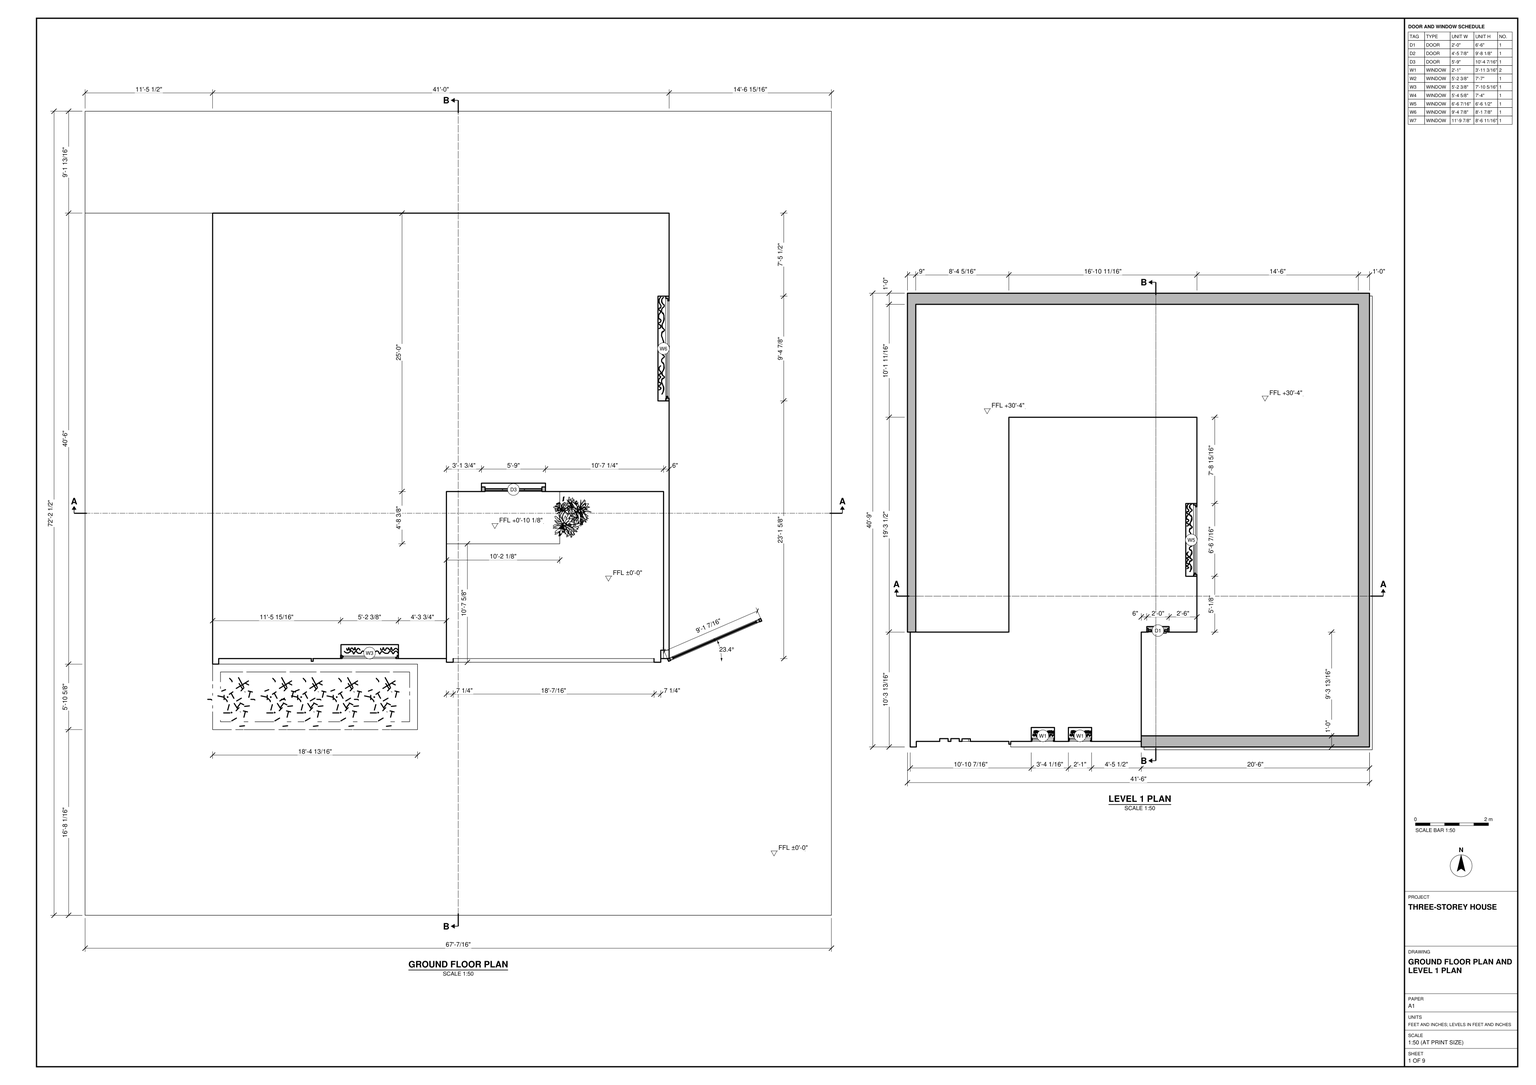
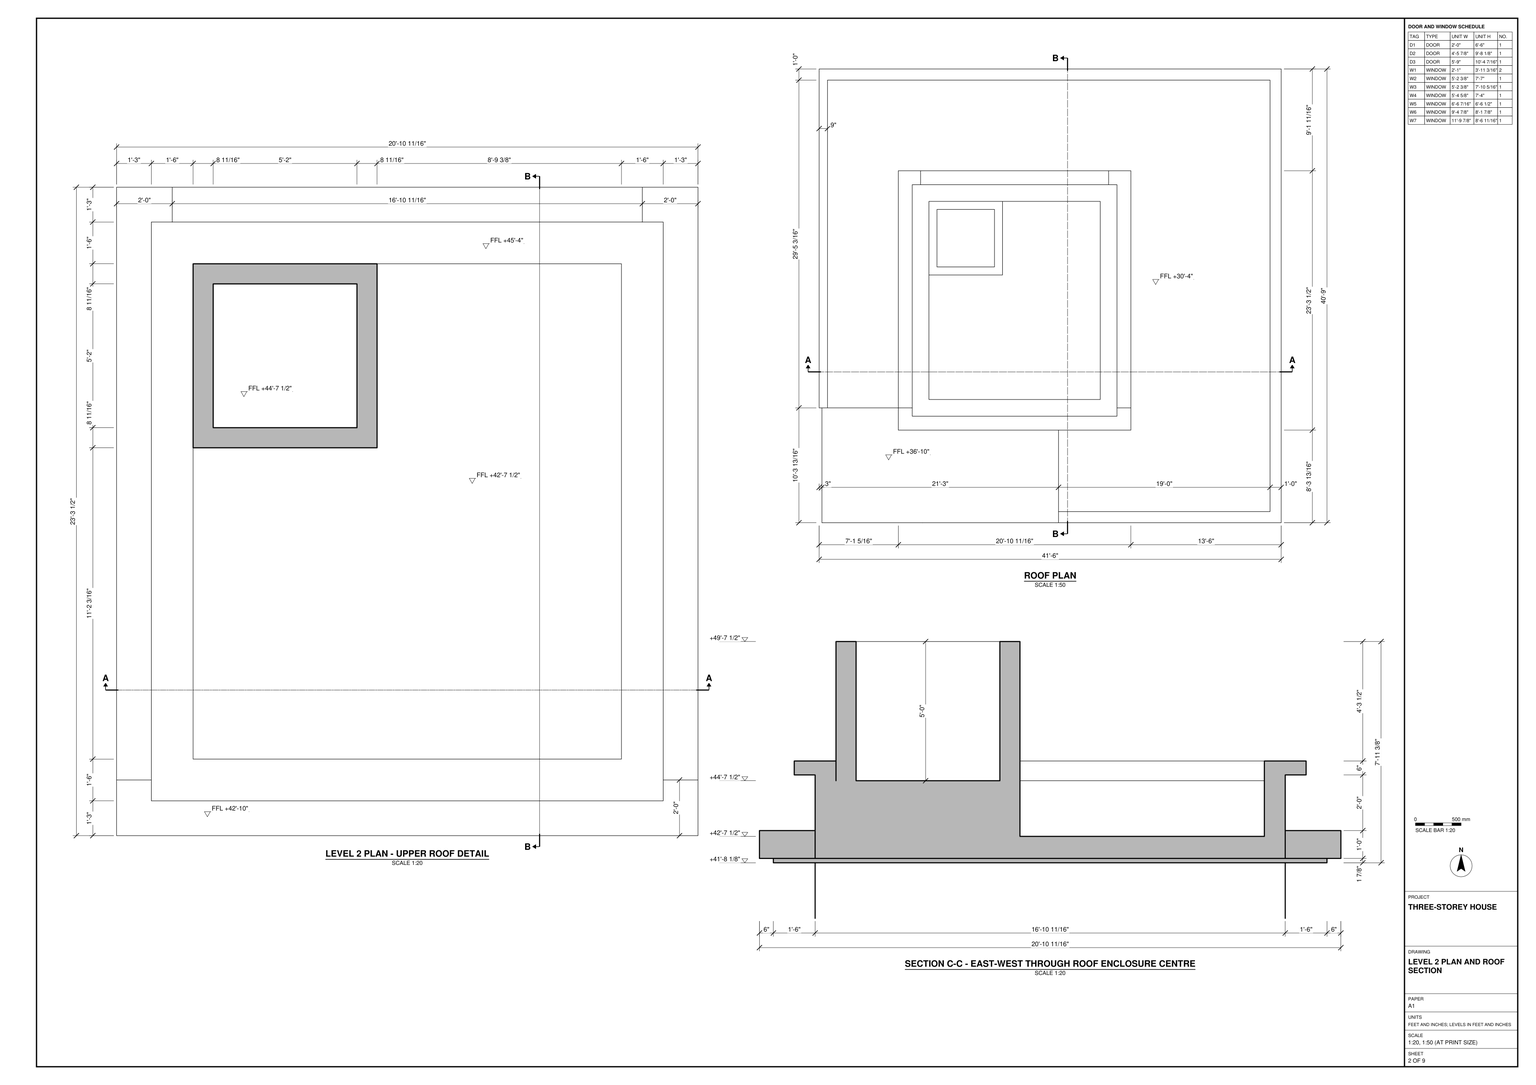
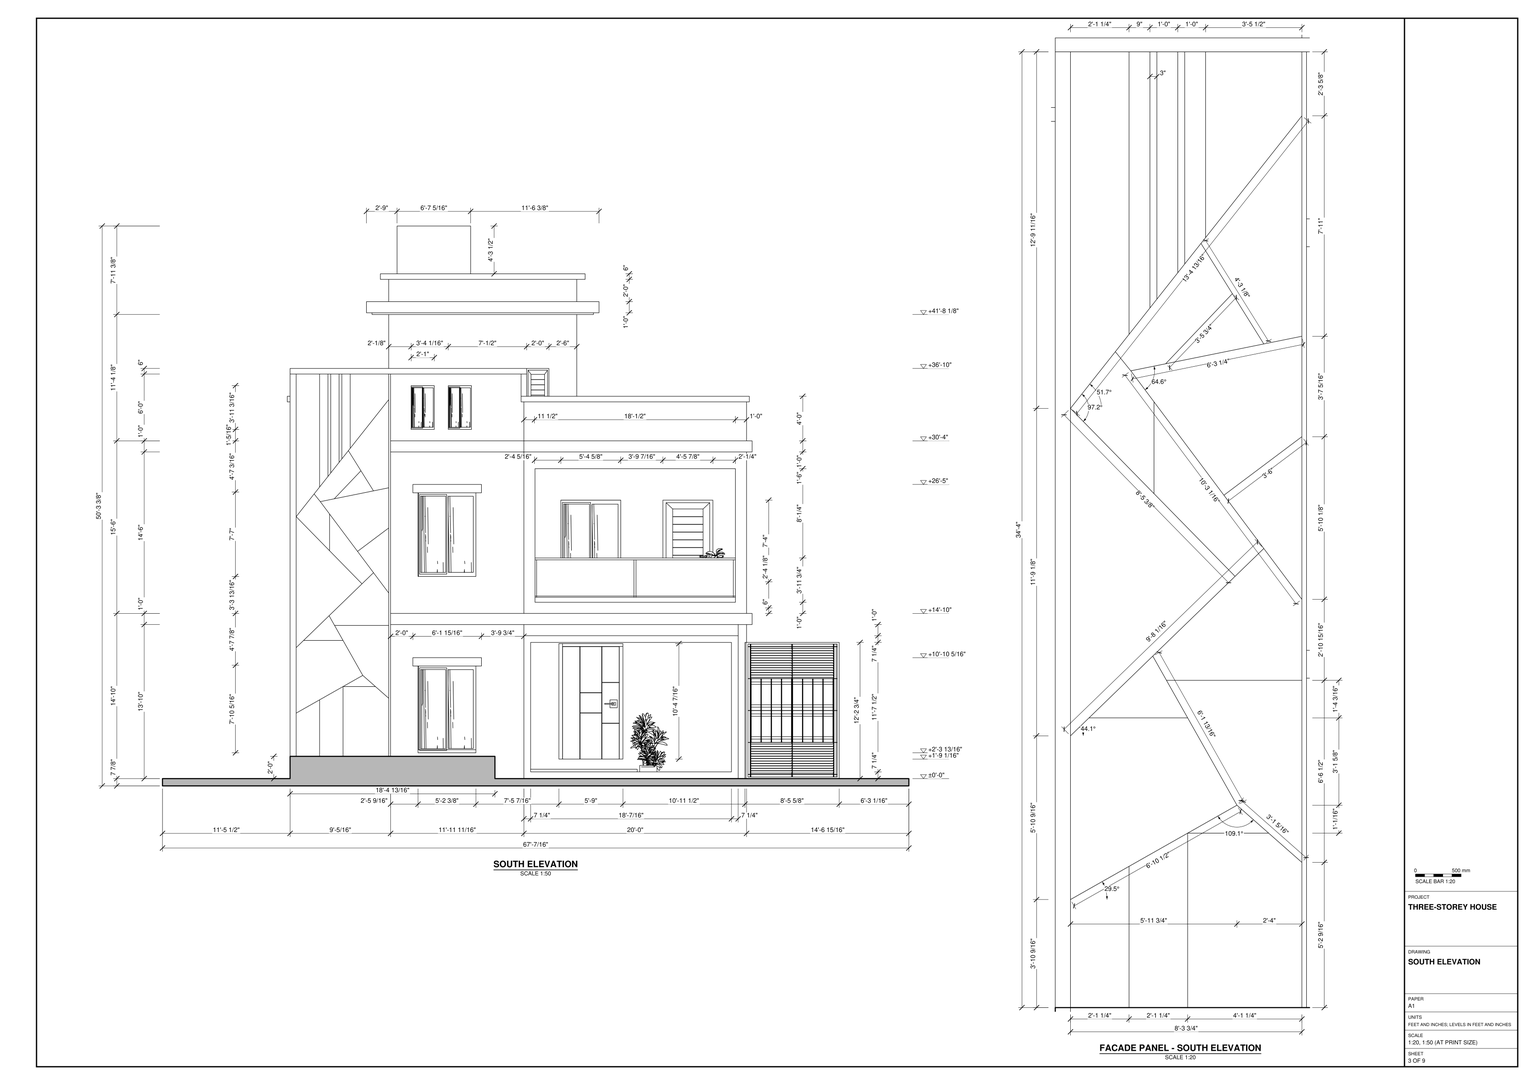
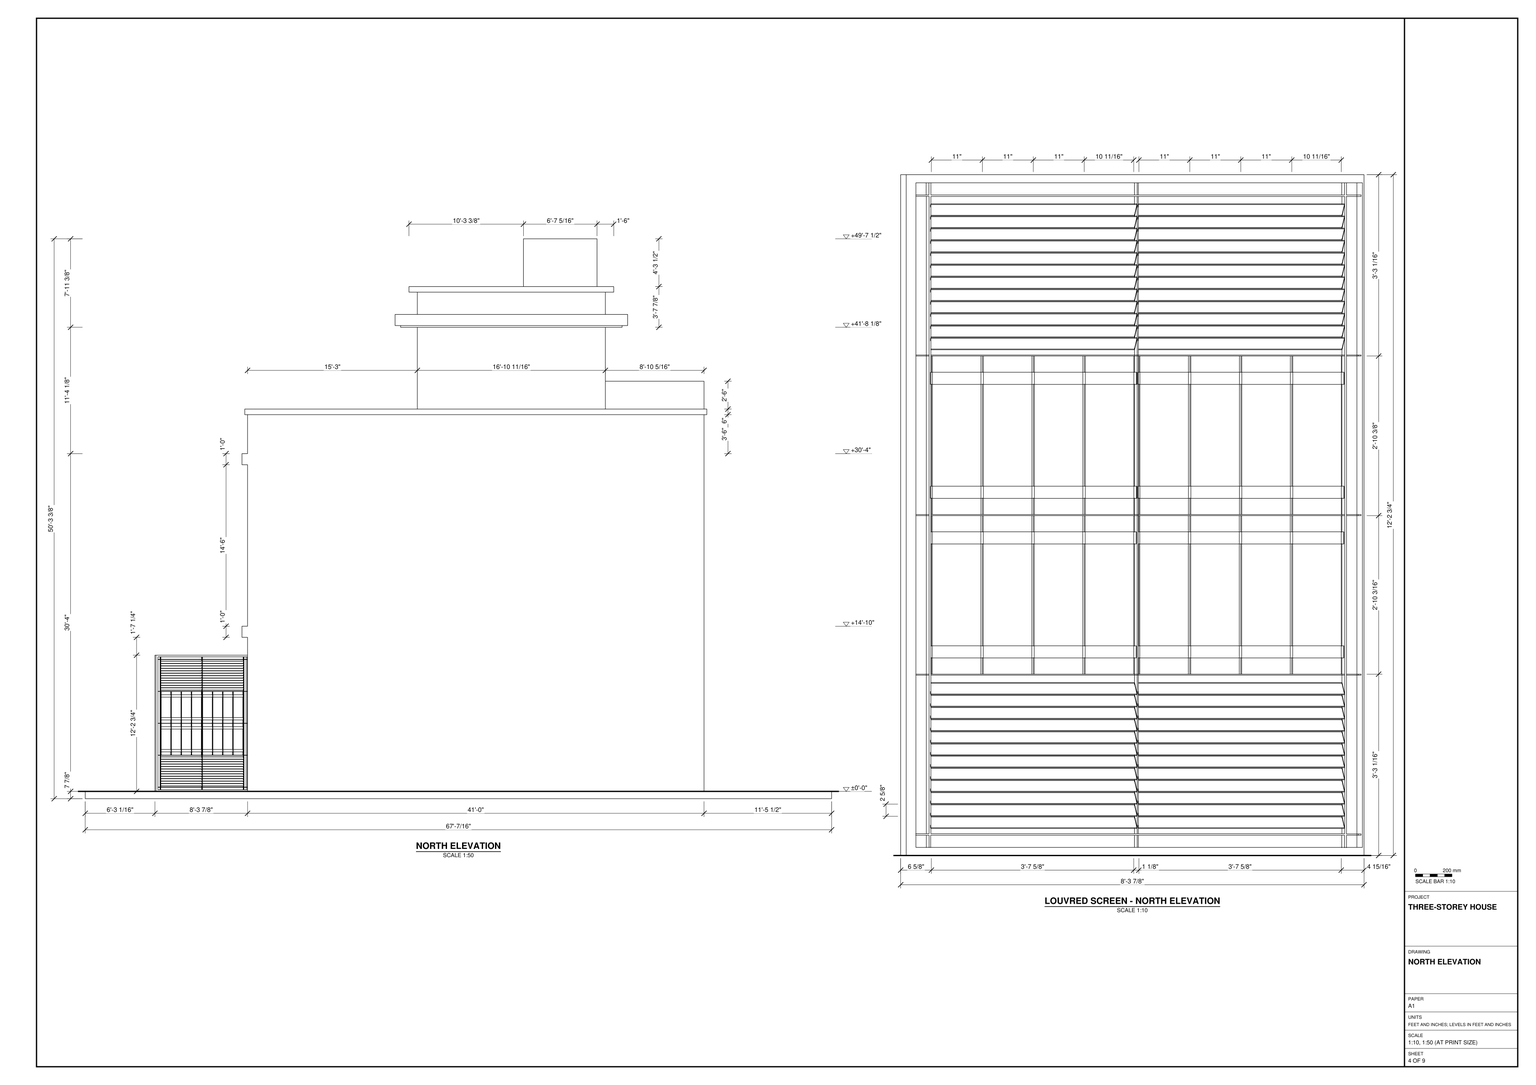
Build the three-storey house in SketchUp from task_files/diagram_01.pdf. Work in feet and inches. Including the rectangular site slab, the overall model must measure 67'-7/16" along X, 72'-2 1/2" along Y and 50'-3 3/8" along Z. Use the storey levels ±0'-0", +30'-4" and +41'-8 1/8" relative to the ground floor.

Use the plans to position the house on the slab and to set out the wall thicknesses, setbacks and openings. On the south elevation, recess the entrance beneath the balcony and fit the balcony with its panelled glass railing. Use the enlarged facade detail to lay out the diagonal and vertical divisions of the tall panel on the left. Set the slatted gate to the right of the entrance at the angle shown in plan. Match the doors and windows to the schedule and elevations. Follow the roof plan and section to model the projecting slab edges, parapets and raised square enclosure. Include stairs, built-in joinery and main furniture where shown.

Keep shell elements such as walls, slabs and roofs, and each furniture or joinery piece, in separate groups or components. Use components for repeated parts. Decor and loose items, including plants, may be any suitable library components. Save one SketchUp model as output_files/three_storey_house_with_its_balcony_and_stepped_roof.skp.

# SketchUp Ruby script. Lengths in inches.
U = 1.inch
M = Sketchup.active_model
def pt(a) = Geom::Point3d.new(a.map { |v| v * U })
def face(e, loops, mat)
  f = e.add_face(loops[0].map { |a| pt(a) })
  loops[1..].each { |l| e.add_face(l.map { |a| pt(a) }).erase! }
  f.material = f.back_material = mat if mat
  f
end
# faces: each face lists its corners as indices into pts; further lists are holes
def faces(e, pts, list, mat = nil) = list.each { |f| face(e, (f[0].is_a?(Array) ? f : [f]).map { |l| l.map { |i| pts[i] } }, mat) }
# xy, xz, yz: faces in a plane at the given z, y or x. An outline is a flat list of corners, or four numbers for a rectangle; further outlines are holes
def ring(l) = l.size == 4 ? [[l[0], l[1]], [l[2], l[1]], [l[2], l[3]], [l[0], l[3]]] : l.each_slice(2).to_a
def flat(e, list, mat, &to3) = list.each { |f| face(e, (f[0].is_a?(Array) ? f : [f]).map { |l| ring(l).map { |u, v| to3.(u, v) } }, mat) }
def xy(e, z, list, mat = nil) = flat(e, list, mat) { |x, y| [x, y, z] }
def xz(e, y, list, mat = nil) = flat(e, list, mat) { |x, z| [x, y, z] }
def yz(e, x, list, mat = nil) = flat(e, list, mat) { |y, z| [x, y, z] }
def lines(e, pts, list) = list.each { |a, b| e.add_line(pt(pts[a]), pt(pts[b])) }
# prism: a flat outline (further loops are holes) pulled along v
def prism(e, loops, v, mat = nil)
  f = face(e, loops, mat); d = Geom::Vector3d.new(v.map { |x| x * U })
  f.pushpull(f.normal.samedirection?(d) ? d.length : -d.length)
end
def box(e, o, s, mat = nil) = prism(e, [[o, [o[0] + s[0], o[1], o[2]], [o[0] + s[0], o[1] + s[1], o[2]], [o[0], o[1] + s[1], o[2]]]], [0, 0, s[2]], mat)
def at(x, y, z, deg = 0) = Geom::Transformation.translation(pt([x, y, z])) * Geom::Transformation.rotation(ORIGIN, Z_AXIS, deg.degrees)
def axes(o, x, y, z) = Geom::Transformation.new([*x, 0, *y, 0, *z, 0, *pt(o).to_a, 1])
def part(name) = M.definitions.add(name)
# library, detail: a bought-in or finely detailed component or shape, given as its bounding box
def library(name, o, s) = part(name).tap { |d| box(d.entities, o, s) }
def detail(e, o, s) = box(e.add_group.entities, o, s)
def put(e, d, t, mat = nil) = e.add_instance(d, t).tap { |i| i.material = mat if mat }
def group(e, t, mat = nil) = e.add_group.tap { |g| g.transformation = t; g.material = mat if mat }.entities
root = M.entities
M.materials.add("Glass Railing Color").color = [198, 198, 198]
M.materials.add("Railing Glass").color = [63, 150, 137]
M.materials["Railing Glass"].alpha = 0.13
M.materials.add("[0030_OldLace]1").color = [221, 214, 201]
M.materials.add("[0035_Tan]").color = [190, 177, 159]
M.materials.add("[0036_BurlyWood]").color = [139, 135, 125]
M.materials.add("[0057_DarkKhaki]1").color = [144, 142, 120]
M.materials.add("[0134_DimGray]").color = [105, 105, 105]
M.materials.add("[0136_Charcoal]").color = [35, 35, 35]
M.materials.add("[Blacktop Old 02]").color = [226, 229, 229]
M.materials.add("[Polished Concrete New]").color = [223, 223, 226]
M.materials.add("[Stone Sandstone Ashlar Light]").color = [206, 178, 128]
M.materials.add("[Wood Veneer 01]").color = [120, 70, 37]
M.materials.add("hymenocallis littoralis").color = [156, 172, 146]
c1 = library("window",[15.03,5.62,-3.05],[94.49,12.1,85.64])
c2 = library("door (4)",[38.93,25.48,0],[40,9.94,82.68])
c3 = library("Door+80x210",[17.88,40.74,0],[31.52,6.14,82.69])
c4 = library("Wade+gate+5.2",[0,-3,0],[48,3,84])
c5 = part("Glass Rail Spacer")
box(c5.entities,[-0.5,-0.25,0],[1,0.5,1],"Glass Railing Color")
c6 = part("Group138\#1")
prism(c6.entities,[[[0.54,0,1.27],[0.38,0,1.39],[0.21,0,1.47],[0.01,0,1.5],[-0.18,0,1.48],[-0.37,0,1.41],[-0.52,0,1.29],[-0.64,0,1.13],[-0.72,0,0.96],[-0.75,0,0.76],[-0.73,0,0.57],[-0.66,0,0.38],[-0.54,0,0.23],[-0.38,0,0.11],[-0.21,0,0.03],[-0.01,0,0],[0.18,0,0.02],[0.37,0,0.09],[0.52,0,0.21],[0.64,0,0.37],[0.72,0,0.54],[0.75,0,0.74],[0.73,0,0.93],[0.66,0,1.12]]],[0,97,0],"Glass Railing Color")
c7 = part("Group141\#1")
prism(c7.entities,[[[0.25,0,5],[0.25,0,4],[-0.25,0,4],[-0.25,0,5],[-0.5,0,5],[-0.5,0,0],[0.5,0,0],[0.5,0,5]]],[0,97,0],"Glass Railing Color")
c8 = part("Group144\#1")
box(c8.entities,[-0.1875,0,0],[0.375,47,30],"Railing Glass")
c9 = part("Group147\#1")
box(c9.entities,[-0.1875,0,0],[0.375,47,30],"Railing Glass")
c10 = part("Glass Railing\#8")
put(c10.entities,c5,at(0,0,4))
put(c10.entities,c5,at(48,0,4))
put(c10.entities,c5,at(96,0,4))
put(c10.entities,c6,at(-0.5,0,34,-90))
put(c10.entities,c7,at(-0.5,0,0,-90))
put(c10.entities,c8,at(0.5,0,4,-90))
put(c10.entities,c9,at(48.5,0,4,-90))
c11 = library("Group_2",[-1.28,-0.39,0],[21.22,20.51,48.44])
c12 = library("plant (7)",[-35.72,-28.42,0],[66.31,67.39,84.38])
c13 = part("Group\#856")
xy(c13.entities,7.38,[[0,0,5.5,15.91]],"hymenocallis littoralis")
p = [[5.5,28.78,0],[5.5,26.79,3.44],[0,26.79,3.44],[0,28.78,0],[0,23.75,6],[5.5,23.75,6],
  [0,15.91,7.38],[5.5,15.91,7.38]]
faces(c13.entities,p,[[0,1,2,3],[4,2,1,5],[6,4,5,7]],"hymenocallis littoralis")
c14 = part("Group\#854")
xy(c14.entities,7.38,[[0,0,5.5,15.91],[0,15.91,5.5,23.87]],"hymenocallis littoralis")
p = [[5.5,31.07,4.3],[5.5,27.74,6.47],[0,27.74,6.47],[0,31.07,4.3],[0,23.87,7.38],[5.5,23.87,7.38]]
faces(c14.entities,p,[[0,1,2,3],[4,2,1,5]],"hymenocallis littoralis")
c15 = part("Group\#857")
xy(c15.entities,7.38,[[0,0,5.6,15.91]],"hymenocallis littoralis")
p = [[5.6,28.78,0],[5.6,26.79,3.44],[0,26.79,3.44],[0,28.78,0],[0,23.75,6],[5.6,23.75,6],
  [0,15.91,7.38],[5.6,15.91,7.38]]
faces(c15.entities,p,[[0,1,2,3],[4,2,1,5],[6,4,5,7]],"hymenocallis littoralis")
c16 = part("Group\#855")
put(c16.entities,c14,axes([6.09,8.57,-0.52],[0.446,0.85617,0.26089],[-0.18444,-0.19731,0.96283],[0.87582,-0.47754,0.0699]))
put(c16.entities,c14,axes([6.29,7.28,-1.71],[0.37058,0.92707,-0.05667],[-0.32382,0.19004,0.99128],[0.87712,-0.32925,0.34964]))
put(c16.entities,c14,axes([11.04,16.14,-0.7],[1,0,0],[0,0.16628,1.02662],[0,-1.18456,0.19186]))
c17 = part("Group\#860")
put(c17.entities,c13,axes([24.57,32.05,-1.76],[0.9552,-0.22102,-0.19681],[0.4036,0.95545,0.88585],[-0.00568,-0.67859,0.7345]))
put(c17.entities,c13,axes([23.95,29.24,-2.4],[0,1,0],[-0.76041,0,0.64945],[0.64945,0,0.76041]))
put(c17.entities,c13,axes([24.22,24.72,-0.48],[-0.70711,0.70711,0],[-0.32757,-0.32757,0.80237],[0.61237,0.61237,0.5]))
put(c17.entities,c14,axes([20.66,37.22,-0.63],[1.12361,0.03262,0.39091],[-0.43499,0.29739,0.78777],[0.09852,-1.27434,0.37535]))
put(c17.entities,c13,axes([28.75,24.45,-2.4],[-1,0,0],[0,-0.76041,0.64945],[0,0.64945,0.76041]))
put(c17.entities,c15,axes([30.4,30.98,-3.7],[0.65676,-0.72002,0.22414],[0.55667,0.66341,0.5],[-0.50871,-0.20361,0.83652]))
put(c17.entities,c15,axes([32.41,29.61,-3.7],[0.04029,-0.97372,0.22414],[0.85287,0.15038,0.5],[-0.52057,0.17102,0.83652]))
put(c17.entities,c13,axes([31.89,25.85,-1.76],[-0.92056,0.33739,-0.19681],[-0.5186,-0.89824,0.88585],[0.08952,0.67268,0.7345]))
put(c17.entities,c13,axes([25.55,34.78,-0.48],[0.86603,0.5,0],[-0.25,0.43301,0.86603],[0.43301,-0.75,0.5]))
put(c17.entities,c15,axes([20.4,16.9375,-8.07],[-0.70711,0.70711,0],[-0.35754,-0.35754,0.65422],[1.3987,1.3987,1.52882]))
put(c17.entities,c13,axes([32.86,34.14,-0.48],[0.76604,-0.64279,0],[0.32139,0.38302,0.86603],[-0.55667,-0.66341,0.5]))
put(c17.entities,c13,axes([27.15,34.7,-0.1],[0.82472,-0.17528,-0.53769],[0.53769,0.53769,0.64945],[0.17528,-0.82472,0.53769]))
put(c17.entities,c13,axes([33.58,28.77,-2.4],[0,-1,0],[0.76041,0,0.64945],[-0.64945,0,0.76041]))
put(c17.entities,c13,axes([26.43,23.87,-2.81],[-0.75126,0.04415,0.65853],[0.53769,-0.53769,0.64945],[0.38276,0.84199,0.3802]))
put(c17.entities,c13,axes([28.78,23.98,-2.4],[-1,0,0],[0,-0.76041,0.64945],[0,0.64945,0.76041]))
put(c17.entities,c13,axes([25.39,25.38,-2.4],[-0.70711,0.70711,0],[-0.53769,-0.53769,0.64945],[0.45923,0.45923,0.76041]))
put(c17.entities,c13,axes([27.32,21.63,-0.1],[-0.45923,0.70711,-0.53769],[-0.76041,0,0.64945],[0.45923,0.70711,0.53769]))
put(c17.entities,c13,axes([25.17,27.625,-1.76],[0.56416,0.80187,-0.19681],[-0.66673,0.66673,0.80532],[0.62659,-0.26057,0.7345]))
put(c17.entities,c15,axes([27.59,27.04,-3.96],[-0.8993,-0.06127,0.43301],[0.2962,-0.8138,0.5],[0.32175,0.57791,0.75]))
put(c17.entities,c15,axes([26.98,24.5,-3.18],[-0.5,0.86603,0],[-0.75,-0.43301,0.5],[0.43301,0.25,0.86603]))
put(c17.entities,c15,axes([24.55,27.74,-3.7],[0.29517,0.92878,0.22414],[-0.85287,0.15038,0.5],[0.43068,-0.33875,0.83652]))
put(c17.entities,c15,axes([24.26,29.8,-3.18],[0.76604,0.64279,0],[-0.47317,0.5639,0.425],[0.32139,-0.38302,0.86603]))
put(c17.entities,c15,axes([25.98,32.46,-3.18],[1,0,0],[0,0.86603,0.5],[0,-0.5,0.86603]))
put(c17.entities,c13,axes([28.78,33.57,-2.4],[1,0,0],[0,0.76041,0.64945],[0,-0.64945,0.76041]))
put(c17.entities,c16,at(14.99,21.38,2.5))
put(c17.entities,c14,axes([34.63,26.34,-1.46],[-0.70089,-0.70877,0.07994],[0.4756,-0.38088,0.79293],[-0.53156,0.59378,0.60405]))
put(c17.entities,c14,axes([28.14,16.92,1.8125],[-1.19719,0.6912,0],[-0.09607,-0.16641,0.94244],[0.68444,1.18549,0.17613]))
put(c17.entities,c14,axes([31.5625,35.84,0.97],[0.66765,-1.1564,0.35779],[0.04445,0.30732,0.91033],[-1.20828,-0.64496,0.17012]))
put(c17.entities,c14,axes([38.94,22.51,0.89],[-0.97932,-0.67164,-0.05202],[0.27787,-0.41401,0.90999],[-0.85985,0.93577,0.32097]))
put(c17.entities,c14,axes([38.44,21.09,1.98],[-1.02864,-0.54856,0.2395],[0.33481,0.06999,0.88388],[-0.77261,1.08328,0.06417]))
put(c17.entities,c15,axes([35.02,30.51,-1.3],[-0.17365,-0.98481,0],[0.60224,-0.10619,0.79122],[-0.7792,0.13739,0.61153]))
put(c17.entities,c15,axes([29.41,22.33,-1.3],[-0.93969,0.34202,0],[-0.20915,-0.57465,0.79122],[0.27061,0.74351,0.61153]))
put(c17.entities,c14,axes([19.64,36,-1.62],[1.18194,0.09546,0.08234],[-0.14377,0.68823,0.76313],[0.21457,-1.1326,0.62386]))
put(c17.entities,c15,axes([24.25,24.14,-1.3],[-0.34202,0.93969,0],[-0.57465,-0.20915,0.79122],[0.74351,0.27061,0.61153]))
put(c17.entities,c15,axes([25.98,34.61,-1.3],[1,0,0],[0,0.61153,0.79122],[0,-0.79122,0.61153]))
put(c17.entities,c15,axes([31.16,34.41,-1.64],[0.56518,-0.80224,-0.19234],[0.73413,0.34233,0.72935],[-0.47639,-0.50772,0.71782]))
put(c17.entities,c15,axes([40.52,26.84,-5.82],[-0.42262,-0.90631,0],[0.48019,-0.22391,0.68552],[-1.43418,0.66877,1.22305]))
put(c17.entities,c13,axes([29.86,38.42,-1.01],[0.89064,-0.37013,0.26413],[-0.03924,0.63286,1.01918],[-0.45353,-0.76487,0.45748]))
put(c17.entities,c13,axes([29.34,22.4,-0.48],[-0.99619,-0.08716,0],[0.04358,-0.4981,0.86603],[-0.07548,0.86273,0.5]))
c18 = part("Group\#858")
xz(c18.entities,10.07,[[9.07,0,10.07,31.01],[0,31.01,0,45.12,20.13,45.12,20.13,31.01,10.07,31.01,10.07,32.58,9.07,32.58,9.07,31.01]],"hymenocallis littoralis")
yz(c18.entities,10.07,[[0,31.01,20.13,45.12]],"hymenocallis littoralis")
p = [[9.57,9.2,0],[10.07,10.07,0],[10.07,10.07,31.01],[10.07,10.07,32.58],[9.57,9.2,32.58]]
faces(c18.entities,p,[[0,1,2,3,4]],"hymenocallis littoralis")
c19 = part("cây lá nắng")
put(c19.entities,c17,axes([49.26,-2.75,0],[0.63109,0.63109,0],[-0.63109,0.63109,0],[0,0,0.935]))
g1 = group(c19.entities,at(26.6,-8.68,0))
put(g1,c13,axes([-4.72,35.73,-1.65],[0.74231,0.46334,-0.18402],[-0.34827,0.85768,0.82827],[0.42467,-0.43184,0.68675]))
put(g1,c13,axes([-3.34,33.57,-2.24],[-0.63109,0.63109,0],[-0.47989,-0.47989,0.60723],[0.40986,0.40986,0.71098]))
put(g1,c13,axes([-0.3125,30.89,-0.45],[-0.8925,0,0],[0,-0.41345,0.75022],[0,0.77293,0.4675]))
put(g1,c14,axes([-10.79,39.66,-0.59],[0.68852,0.72969,0.3655],[-0.4622,-0.08684,0.73657],[0.86641,-0.74205,0.35095]))
put(g1,c13,axes([2.71,33.57,-2.24],[-0.63109,-0.63109,0],[0.47989,-0.47989,0.60723],[-0.40986,0.40986,0.71098]))
put(g1,c15,axes([-0.37,38.74,-3.46],[0.86887,-0.03992,0.20957],[-0.06737,0.76999,0.4675],[-0.19255,-0.44954,0.78214]))
put(g1,c15,axes([1.76,39.14,-3.46],[0.63993,-0.58908,0.20957],[0.44333,0.63315,0.4675],[-0.43646,-0.2206,0.78214]))
put(g1,c13,axes([3.81,36.4375,-1.65],[-0.79389,-0.36803,-0.18402],[0.23959,-0.89415,0.82827],[-0.36803,0.48102,0.68675]))
put(g1,c13,axes([-5.83,38.07,-0.45],[0.231,0.86209,0],[-0.43104,0.1155,0.80973],[0.74659,-0.20005,0.4675]))
put(g1,c15,axes([2.18,23.5625,-7.55],[-0.8925,0,0],[0,-0.45128,0.6117],[0,1.76542,1.42944]))
put(g1,c13,axes([-0.8125,42.28,-0.45],[0.8891,0.07779,0],[-0.03889,0.44455,0.80973],[0.06737,-0.76999,0.4675]))
put(g1,c13,axes([-4.76,39.03,-0.09],[0.63109,0.40986,-0.50274],[0,0.67866,0.60723],[0.63109,-0.40986,0.50274]))
put(g1,c13,axes([3.03,39.35,-2.24],[0.63109,-0.63109,0],[0.47989,0.47989,0.60723],[-0.40986,-0.40986,0.71098]))
put(g1,c13,axes([1.61,31.74,-2.625],[-0.50198,-0.44625,0.61573],[0.67866,0,0.60723],[-0.28982,0.77293,0.35549]))
put(g1,c13,axes([3.03,33.3,-2.24],[-0.63109,-0.63109,0],[0.47989,-0.47989,0.60723],[-0.40986,0.40986,0.71098]))
put(g1,c13,axes([0.01,32.04,-2.24],[-0.8925,0,0],[0,-0.67866,0.60723],[0,0.57963,0.71098]))
put(g1,c13,axes([3.59,30.89,-0.09],[-0.73607,0.15643,-0.50274],[-0.47989,-0.47989,0.60723],[-0.15643,0.73607,0.50274]))
put(g1,c13,axes([-1.55,33.32,-1.65],[-0.15002,0.86209,-0.18402],[-0.84154,0,0.75297],[0.55988,0.231,0.68675]))
put(g1,c15,axes([0.35,34.48,-3.71],[-0.52887,-0.60621,0.40487],[0.70051,-0.32665,0.4675],[-0.16166,0.56777,0.70125]))
put(g1,c15,axes([2.61,39.13,-1.74],[-0.86209,0.231,0],[-0.23031,-0.85954,0.15531],[0.03162,0.11799,0.91645]))
put(g1,c15,axes([-2.02,33,-3.46],[-0.39986,0.77243,0.20957],[-0.63315,-0.44333,0.4675],[0.48558,0.05802,0.78214]))
put(g1,c15,axes([-3.49,34.12,-2.97],[0.07779,0.8891,0],[-0.65449,0.05726,0.39737],[0.44455,-0.03889,0.80973]))
put(g1,c15,axes([-4.09,36.88,-2.97],[0.63109,0.63109,0],[-0.54654,0.54654,0.4675],[0.31555,-0.31555,0.80973]))
put(g1,c13,axes([-3.02,39.35,-2.24],[0.63109,0.63109,0],[-0.47989,0.47989,0.60723],[0.40986,-0.40986,0.71098]))
put(g1,c16,axes([-4.03,22.95,2.33],[0.63109,0.63109,0],[-0.63109,0.63109,0],[0,0,0.935]))
put(g1,c14,axes([5.24,38.48,-1.37],[0.00497,-0.88963,0.07474],[0.54052,0.05978,0.74139],[-0.71019,0.03927,0.56479]))
put(g1,c14,axes([7.08,28.4375,1.7],[-1.19175,-0.31933,0],[0.04439,-0.16565,0.88118],[-0.31621,1.1801,0.16468]))
put(g1,c14,axes([-2.7,42.54,0.91],[1.15114,-0.30845,0.33454],[-0.1659,0.22199,0.85115],[-0.3555,-1.16957,0.15907]))
put(g1,c14,axes([10.37,38.78,0.83],[-0.19417,-1.04191,-0.04864],[0.43664,-0.08592,0.85084],[-1.1332,0.04791,0.30011]))
put(g1,c14,axes([10.95,37.5625,1.85],[-0.30298,-0.99536,0.22393],[0.16713,0.25547,0.82643],[-1.17124,0.19607,0.06]))
put(g1,c15,axes([2.84,41.36,-1.22],[0.51192,-0.73109,0],[0.44708,0.31305,0.73979],[-0.57846,-0.40504,0.57178]))
put(g1,c15,axes([4.47,32.65,-1.22],[-0.80888,-0.37719,0],[0.23066,-0.49465,0.73979],[-0.29844,0.64,0.57178]))
put(g1,c14,axes([-10.32,35.12,-1.51],[0.68567,0.80616,0.07699],[-0.52507,0.3436,0.71352],[0.85019,-0.57936,0.58331]))
put(g1,c15,axes([0.07,30.54,-1.22],[-0.80888,0.37719,0],[-0.23066,-0.49465,0.73979],[0.29844,0.64,0.57178]))
put(g1,c15,axes([-5.45,38.24,-1.22],[0.63109,0.63109,0],[-0.38593,0.38593,0.73979],[0.49934,-0.49934,0.57178]))
put(g1,c15,axes([-2.05,41.38,-1.53],[0.86296,-0.14961,-0.17984],[0.24726,0.67935,0.68194],[0.01977,-0.62107,0.67116]))
put(g1,c15,axes([8.63,42.51,-5.4375],[0.30525,-0.83868,0],[0.44435,0.16173,0.64096],[-1.32716,-0.48305,1.14356]))
put(g1,c13,axes([-5.4,43.09,-0.94],[0.79566,0.32849,0.24696],[-0.42416,0.37462,0.95293],[0.19648,-0.76892,0.42774]))
put(g1,c13,axes([4.38,32.65,-0.45],[-0.57369,-0.68369,0],[0.34185,-0.28684,0.80973],[-0.5921,0.49683,0.4675]))
put(g1,c15,axes([-2,33.84,-0.15],[-0.24601,0.85793,0],[-0.85539,-0.24528,0.15531],[0.11742,0.03367,0.91645]))
put(g1,c15,axes([0.17,30.83,-4.47],[-0.24601,0.85793,0],[-0.85539,-0.24528,0.15531],[0.11742,0.03367,0.91645]))
put(g1,c15,axes([-1.97,32.18,-4.47],[0.58524,0.67383,0],[-0.67184,0.58351,0.15531],[0.09222,-0.0801,0.91645]))
put(g1,c15,axes([-2,34.71,-4.47],[0.88392,-0.12346,0],[0.12309,0.88131,0.15531],[-0.0169,-0.12098,0.91645]))
put(g1,c15,axes([0.11,36.12,-4.47],[0.37822,-0.8084,0],[0.80601,0.37711,0.15531],[-0.11064,-0.05177,0.91645]))
put(c19.entities,c18,axes([29.71,14.29,6.94],[0.425,0.73612,0],[-0.6771,0.39092,-0.33349],[-0.26859,0.15507,0.72712]))
put(c19.entities,c18,axes([42.0625,26.12,6.94],[0.85,0,0],[0,0.78185,-0.33349],[0,0.33349,0.78185]))
put(c19.entities,c17,axes([7.3125,23.0625,0],[0.8925,0,0],[0,0.8925,0],[0,0,0.935]))
put(c19.entities,c18,axes([24.4375,40.23,2.05],[0.85,0,0],[0,0.85,0],[0,0,0.85]))
c20 = part("Planting+101")
put(c20.entities,c19,axes([21.34,32.96,-4.59],[0,-0.71,0],[-0.71,0,0],[0,0,0.71]))
xy(root,6.125,[[[0,0,804.4375,866.5],[620.5,276.6875,629.5,285.6875]],[620.5,276.6875,623.5,285.6875],[623.5,276.6875,629.5,285.6875]])
xy(root,13.99,[[145.98,208.54,349.84,262.21]],"[0030_OldLace]1")
xy(root,13.99,[[0,0,804.4375,0,804.4375,866.5,0,866.5,0,756.6875,629.5,756.6875,629.5,276.6875,620.5,276.6875,620.5,272.6875,389.5,272.6875,389.5,276.6875,245.83,276.6875,245.83,273.6875,243.83,273.6875,243.83,276.6875,144.0625,276.6875,144.0625,270.6875,358.3125,270.6875,358.3125,200.0625,137.5,200.0625,137.5,756.6875,0,756.6875],[389.5,272.6875,620.5,272.6875,620.5,276.6875,623.5,276.6875,623.5,456.6875,511.625,456.6875,511.625,400.3125,389.5,400.3125]],"[Polished Concrete New]")
xy(root,21.26,[[396.77,272.6875,613.23,276.6875]],"[0136_Charcoal]")
xy(root,24.11,[[389.5,400.3125,511.625,456.6875]],"[Wood Veneer 01]")
xy(root,35.04,[[427.24,456.6875,496.24,465.6875]])
xy(root,37.99,[[[137.5,200.0625,358.3125,270.6875],[145.98,208.54,349.84,262.21]]],"[0030_OldLace]1")
xy(root,39.84,[[617.5,554.34,629.5,667.21]])
xy(root,45.13,[[275.84,276.6875,337.77,291.6875]],"[0134_DimGray]")
xy(root,91,[[623.5,285.6875,629.5,382.5]],"[0030_OldLace]1")
xy(root,135.32,[[269.84,270.6875,269.84,276.6875,275.84,276.6875,275.84,291.6875,337.77,291.6875,337.77,276.6875,343.77,276.6875,343.77,270.6875]],"[0030_OldLace]1")
xy(root,137.65,[[617.5,554.34,629.5,667.21]])
xy(root,144.32,[[269.84,270.6875,343.77,276.6875]],"[0030_OldLace]1")
xy(root,159.48,[[427.24,456.6875,496.24,465.6875]])
xy(root,160.73,[[396.77,272.6875,613.23,276.6875]],"[0136_Charcoal]")
xy(root,168,[[389.5,276.6875,620.5,282.6875],[623.5,285.6875,629.5,382.5]],"[0030_OldLace]1")
xy(root,168,[[389.5,272.6875,620.5,276.6875]],"[0136_Charcoal]")
xy(root,180,[[389.5,282.6875,389.5,456.6875,623.5,456.6875,623.5,285.6875,620.5,285.6875,620.5,282.6875]],"[0030_OldLace]1")
xy(root,180,[[245.83,267.6875,389.5,276.6875],[389.5,267.6875,389.5,276.6875,629.5,276.6875,629.5,456.6875,635.5,456.6875,635.5,267.6875],[629.5,456.6875,635.5,756.6875]],"[0057_DarkKhaki]1")
xy(root,192,[[245.83,267.6875,635.5,267.6875,635.5,273.6875,389.5,273.6875,389.5,276.6875,245.83,276.6875],[629.5,273.6875,635.5,756.6875]],"[0057_DarkKhaki]1")
xy(root,198,[[395.5,282.6875,617.5,282.6875,617.5,336.6875,593.22,336.6875,593.22,345.6875,539.35,345.6875,539.35,336.6875,395.5,336.6875]],"[0030_OldLace]1")
xy(root,204,[[401.5,273.6875,617.5,282.6875],[617.5,282.6875,629.5,336.6875]],"[0030_OldLace]1")
xy(root,226.11,[[429.31,336.6875,493.93,351.6875]],"[0134_DimGray]")
xy(root,228.88,[[617.5,391.65,629.5,533.53]])
xy(root,231.82,[[275.84,276.6875,337.77,291.6875]],"[0134_DimGray]")
xy(root,314.11,[[539.35,336.6875,593.22,345.6875]])
xy(root,314.11,[[429.31,336.6875,493.93,351.6875]],"[0134_DimGray]")
xy(root,322,[[269.84,270.6875,269.84,276.6875,275.84,276.6875,275.84,291.6875,337.77,291.6875,337.77,276.6875,343.77,276.6875,343.77,270.6875]],"[0030_OldLace]1")
xy(root,331,[[269.84,270.6875,343.77,276.6875]],"[0030_OldLace]1")
xy(root,331.5,[[617.5,391.65,629.5,533.53]])
xy(root,348,[[401.5,273.6875,617.5,282.6875]],"[0030_OldLace]1")
xy(root,354,[[395.5,282.6875,629.5,336.6875]],"[0030_OldLace]1")
xy(root,366,[[389.5,267.6875,389.5,273.6875,629.5,273.6875,629.5,756.6875,635.5,756.6875,635.5,267.6875],[245.83,270.6875,389.5,276.6875]],"[0057_DarkKhaki]1")
xy(root,378,[[386.5,282.6875,620.5,282.6875,620.5,747.6875,143.5,747.6875,143.5,394.48,243.83,394.48,243.83,626,446.5,626,446.5,394.48,416.5,394.48,416.5,400.48,392.5,400.48,392.5,394.48,386.5,394.48]],"[0030_OldLace]1")
xy(root,378,[[389.5,267.6875,635.5,267.6875,635.5,756.6875,629.5,756.6875,629.5,273.6875,389.5,273.6875],[245.83,270.6875,389.5,276.6875]],"[0057_DarkKhaki]1")
xy(root,390.3,[[267.95,276.6875,292.95,291.6875],[308.01,276.6875,333.01,291.6875]],"[0134_DimGray]")
xy(root,398.3,[[434.5,454.61,446.5,533.05]])
xy(root,420,[[386.5,276.6875,389.5,282.6875]])
xy(root,420,[[386.5,270.6875,386.5,276.6875,389.5,276.6875,389.5,273.6875,629.5,273.6875,629.5,756.6875,137.5,756.6875,137.5,394.48,134.5,394.48,134.5,759.6875,632.5,759.6875,632.5,270.6875]],"[0057_DarkKhaki]1")
xy(root,426,[[386.5,270.6875,632.5,270.6875,632.5,759.6875,134.5,759.6875,134.5,394.48,143.5,394.48,143.5,747.6875,620.5,747.6875,620.5,282.6875,386.5,282.6875]],"[0057_DarkKhaki]1")
xy(root,437.42,[[267.95,276.6875,292.95,291.6875],[308.01,276.6875,333.01,291.6875]],"[0134_DimGray]")
xy(root,450,[[144.0625,270.6875,144.0625,276.6875,169.32,276.6875,169.32,279.6875,178.32,279.6875,178.32,276.6875,181.32,276.6875,181.32,279.6875,190.32,279.6875,190.32,276.6875,193.32,276.6875,193.32,279.5,202.32,279.5,202.32,276.6875,243.83,276.6875,243.83,270.6875],[243.83,270.6875,245.83,273.6875],[245.83,270.6875,245.83,276.6875,386.5,276.6875,386.5,394.48,392.5,394.48,392.5,270.6875]],"[0057_DarkKhaki]1")
xy(root,456,[[392.5,394.48,416.5,400.48]])
xy(root,456,[[137.5,270.6875,392.5,394.48]],"[0057_DarkKhaki]1")
xy(root,476.74,[[434.5,454.61,446.5,533.05]])
xy(root,514.125,[[243.83,394.48,446.5,626]])
xy(root,514.125,[[[225.83,376.48,464.5,644],[243.83,394.48,446.5,626]]],"[0030_OldLace]1")
xy(root,516,[[225.83,376.48,243.83,644],[243.83,376.48,464.5,394.48],[243.83,394.48,446.5,626],[446.5,394.48,464.5,626],[243.83,626,464.5,644]])
xy(root,516,[[[219.83,370.48,470.5,650],[225.83,376.48,464.5,644]]],"[0030_OldLace]1")
xy(root,525.5,[[252.83,403.48,437.5,403.48,437.5,617,332.14,617,332.14,537.6875,252.83,537.6875]],"[0030_OldLace]1")
xy(root,528,[[219.83,370.48,470.5,394.48],[219.83,394.48,243.83,650],[446.5,394.48,470.5,650],[243.83,626,446.5,650]],"[0030_OldLace]1")
xy(root,549.5,[[261.49,546.35,323.48,608.34]])
xy(root,552,[[[234.83,385.48,455.5,635],[243.83,394.48,446.5,626]]],"[0036_BurlyWood]")
xy(root,558,[[[234.83,385.48,455.5,635],[252.83,403.48,437.5,617]]],"[0036_BurlyWood]")
xy(root,609.5,[[[252.83,537.6875,332.14,617],[261.49,546.35,323.48,608.34]]],"[0035_Tan]")
xz(root,0,[[0,6.125,804.4375,13.99]],"[Blacktop Old 02]")
xz(root,200.0625,[[137.5,13.99,358.3125,37.99]],"[0030_OldLace]1")
xz(root,208.54,[[145.98,13.99,349.84,37.99]],"[0030_OldLace]1")
xz(root,262.21,[[145.98,13.99,349.84,37.99]],"[0030_OldLace]1")
xz(root,267.6875,[[245.83,180,635.5,192],[389.5,366,635.5,378]],"[0057_DarkKhaki]1")
xz(root,270.6875,[[144.0625,13.99,358.3125,37.99]])
xz(root,270.6875,[[269.84,135.32,343.77,144.32],[269.84,322,343.77,331]],"[0030_OldLace]1")
xz(root,270.6875,[[137.5,37.99,144.0625,450],[245.83,366,389.5,378],[386.5,420,632.5,426],[137.5,450,392.5,456]],"[0057_DarkKhaki]1")
xz(root,272.6875,[[[389.5,13.99,620.5,168],[396.77,21.26,613.23,160.73]]],"[0136_Charcoal]")
xz(root,273.6875,[[[389.5,192,629.5,366],[401.5,204,617.5,348]],[389.5,378,629.5,420]],"[0030_OldLace]1")
xz(root,273.6875,[[243.83,13.99,245.83,450]],"[0057_DarkKhaki]1")
xz(root,276.6875,[[620.5,6.125,623.5,13.99],[623.5,6.125,629.5,13.99]])
xz(root,276.6875,[[144.0625,13.99,169.32,13.99,169.32,98.88,144.0625,84.57],[169.32,13.99,194.58,13.99,194.58,113.1875,169.32,98.88],[194.58,13.99,243.83,13.99,243.83,100.58,229.51,113.1875,194.58,113.1875],[620.5,13.99,629.5,180],[243.83,100.58,243.83,179.06,185.45,179.06,194.58,162.88,215.84,125.23,229.51,113.1875],
  [144.0625,155.14,152.05,162.88,179.54,189.52,215.02,223.9,180.08,259.55,144.0625,296.29],[389.5,168,620.5,180],[185.45,179.06,243.83,179.06,243.83,213.98,227.41,235.9,215.02,223.9,179.54,189.52],[243.83,213.98,243.83,284.1,210.22,258.87,227.41,235.9],[215.02,223.9,227.41,235.9,210.22,258.87,180.08,299.12,180.08,259.55],
  [210.22,258.87,243.83,284.1,243.83,327.39,227.41,324.07,185.09,315.52,170.07,312.48,180.08,299.12],[144.0625,296.29,163.41,320.74,169.32,328.22,169.32,450,144.0625,450],[170.07,312.48,185.09,315.52,213.87,345.74,200.32,367.41,193.32,358.56,190.32,354.77,181.32,343.39,178.32,339.6,169.32,328.22,163.41,320.74],[227.41,324.07,243.83,327.39,243.83,422.39,202.32,369.93,200.32,367.41,213.87,345.74],[178.32,339.6,181.32,343.39,181.32,450,178.32,450],
  [190.32,354.77,193.32,358.56,193.32,450,190.32,450],[202.32,369.93,243.83,422.39,243.83,450,202.32,450],[[245.83,378,389.5,378,389.5,420,386.5,420,386.5,450,245.83,450],[267.95,390.3,292.95,437.42],[308.01,390.3,333.01,437.42]]],"[0030_OldLace]1")
xz(root,276.6875,[[[245.83,13.99,389.5,180],[275.84,45.13,275.84,135.32,269.84,135.32,269.84,144.32,343.77,144.32,343.77,135.32,337.77,135.32,337.77,45.13]],[144.0625,84.57,169.32,98.88,194.58,113.1875,215.84,125.23,194.58,162.88,152.05,162.88,144.0625,155.14]],"[0035_Tan]")
xz(root,276.6875,[[[245.83,192,389.5,366],[275.84,231.82,275.84,322,269.84,322,269.84,331,343.77,331,343.77,322,337.77,322,337.77,231.82]]],"[0036_BurlyWood]")
xz(root,276.6875,[[194.58,113.1875,229.51,113.1875,215.84,125.23],[152.05,162.88,194.58,162.88,185.45,179.06,179.54,189.52],[180.08,259.55,180.08,299.12,170.07,312.48,163.41,320.74,144.0625,296.29],[185.09,315.52,227.41,324.07,213.87,345.74]],"[0057_DarkKhaki]1")
xz(root,279.5,[[193.32,358.56,200.32,367.41,202.32,369.93,202.32,450,193.32,450]],"[0057_DarkKhaki]1")
xz(root,279.6875,[[169.32,328.22,178.32,339.6,178.32,450,169.32,450],[181.32,343.39,190.32,354.77,190.32,450,181.32,450]],"[0057_DarkKhaki]1")
xz(root,282.6875,[[389.5,168,620.5,180],[395.5,198,617.5,204],[395.5,204,401.5,354],[617.5,204,629.5,354],[401.5,348,617.5,354],
  [386.5,378,398.5,426],[398.5,378,620.5,426]],"[0030_OldLace]1")
xz(root,285.6875,[[623.5,6.125,629.5,13.99]])
xz(root,285.6875,[[620.5,6.125,623.5,180],[623.5,91,629.5,168]],"[0030_OldLace]1")
xz(root,291.6875,[[275.84,45.13,337.77,135.32],[275.84,231.82,337.77,322],[267.95,390.3,292.95,437.42],[308.01,390.3,333.01,437.42]],"[0134_DimGray]")
xz(root,336.6875,[[[395.5,198,539.35,198,539.35,314.11,593.22,314.11,593.22,198,617.5,198,617.5,204,629.5,204,629.5,354,395.5,354],[429.31,226.11,493.93,314.11]]],"[0030_OldLace]1")
xz(root,345.6875,[[539.35,198,593.22,314.11]])
xz(root,351.6875,[[429.31,226.11,493.93,314.11]],"[0134_DimGray]")
xz(root,370.48,[[219.83,516,470.5,528]],"[0030_OldLace]1")
xz(root,376.48,[[225.83,514.125,464.5,516]],"[0030_OldLace]1")
xz(root,382.5,[[623.5,91,629.5,168]],"[0030_OldLace]1")
xz(root,385.48,[[234.83,552,455.5,558]],"[0036_BurlyWood]")
xz(root,391.65,[[617.5,228.88,629.5,331.5]])
xz(root,394.48,[[137.5,420,143.5,426],[243.83,516,446.5,528]])
xz(root,394.48,[[143.5,378,143.5,426,137.5,426,137.5,456,243.83,456,243.83,378],[416.5,378,446.5,378,446.5,514.125,243.83,514.125,243.83,456,416.5,456],[386.5,378,392.5,450],[134.5,420,137.5,426]],"[0030_OldLace]1")
xz(root,394.48,[[243.83,528,446.5,552]],"[0036_BurlyWood]")
xz(root,400.3125,[[389.5,13.99,511.625,24.11]],"[Wood Veneer 01]")
xz(root,400.48,[[392.5,378,416.5,456]])
xz(root,403.48,[[252.83,525.5,437.5,549.5],[252.83,549.5,437.5,558]],"[0036_BurlyWood]")
xz(root,454.61,[[434.5,398.3,446.5,476.74]])
xz(root,456.6875,[[[511.625,13.99,623.5,13.99,623.5,180,389.5,180,389.5,24.11,511.625,24.11],[427.24,35.04,496.24,159.48]]],"[0030_OldLace]1")
xz(root,465.6875,[[427.24,35.04,496.24,159.48]])
xz(root,533.05,[[434.5,398.3,446.5,476.74]])
xz(root,533.53,[[617.5,228.88,629.5,331.5]])
xz(root,537.6875,[[252.83,525.5,332.14,609.5]],"[0035_Tan]")
xz(root,546.35,[[261.49,549.5,323.48,609.5]],"[0035_Tan]")
xz(root,554.34,[[617.5,39.84,629.5,137.65]])
xz(root,608.34,[[261.49,549.5,323.48,609.5]],"[0035_Tan]")
xz(root,617,[[252.83,549.5,332.14,558]])
xz(root,617,[[252.83,558,332.14,609.5]],"[0035_Tan]")
xz(root,617,[[332.14,525.5,437.5,549.5],[332.14,549.5,437.5,558]],"[0036_BurlyWood]")
xz(root,626,[[243.83,516,446.5,528]])
xz(root,626,[[243.83,378,446.5,514.125]],"[0030_OldLace]1")
xz(root,626,[[243.83,528,446.5,552]],"[0036_BurlyWood]")
xz(root,635,[[234.83,552,455.5,558]],"[0036_BurlyWood]")
xz(root,644,[[225.83,514.125,464.5,516]],"[0030_OldLace]1")
xz(root,650,[[219.83,516,470.5,528]],"[0030_OldLace]1")
xz(root,667.21,[[617.5,39.84,629.5,137.65]])
xz(root,747.6875,[[143.5,378,398.5,378,398.5,426,389.5,426,389.5,420,143.5,420],[398.5,378,620.5,426],[143.5,420,389.5,426]],"[0030_OldLace]1")
xz(root,756.6875,[[0,6.125,137.5,13.99],[137.5,6.125,629.5,13.99]])
xz(root,756.6875,[[137.5,13.99,137.5,420,629.5,420,629.5,378,635.5,378,635.5,366,629.5,366,629.5,192,635.5,192,635.5,180,629.5,180,629.5,13.99]],"[0030_OldLace]1")
xz(root,759.6875,[[134.5,420,632.5,426]],"[0030_OldLace]1")
xz(root,866.5,[[0,6.125,804.4375,13.99]],"[Blacktop Old 02]")
yz(root,0,[[0,6.125,756.6875,13.99],[756.6875,6.125,866.5,13.99]],"[Blacktop Old 02]")
yz(root,134.5,[[394.48,420,759.6875,426]],"[0030_OldLace]1")
yz(root,137.5,[[200.0625,13.99,270.6875,37.99],[270.6875,13.99,270.6875,456,394.48,456,394.48,378,756.6875,378,756.6875,13.99],[394.48,378,756.6875,420]],"[0030_OldLace]1")
yz(root,143.5,[[394.48,378,747.6875,420],[394.48,420,747.6875,426]],"[0030_OldLace]1")
yz(root,144.0625,[[270.6875,13.99,276.6875,450]],"[0057_DarkKhaki]1")
yz(root,145.98,[[208.54,13.99,262.21,37.99]],"[0030_OldLace]1")
yz(root,169.32,[[276.6875,328.22,279.6875,450]],"[0057_DarkKhaki]1")
yz(root,178.32,[[276.6875,339.6,279.6875,450]],"[0030_OldLace]1")
yz(root,181.32,[[276.6875,343.39,279.6875,450]],"[0030_OldLace]1")
yz(root,190.32,[[276.6875,354.77,279.6875,450]],"[0030_OldLace]1")
yz(root,193.32,[[276.6875,358.56,279.5,450]],"[0030_OldLace]1")
yz(root,202.32,[[276.6875,369.93,279.5,450]],"[0057_DarkKhaki]1")
yz(root,219.83,[[370.48,516,650,528]],"[0030_OldLace]1")
yz(root,225.83,[[376.48,514.125,644,516]],"[0030_OldLace]1")
yz(root,234.83,[[385.48,552,635,558]],"[0036_BurlyWood]")
yz(root,243.83,[[394.48,516,626,528]])
yz(root,243.83,[[394.48,378,626,514.125]],"[0030_OldLace]1")
yz(root,243.83,[[394.48,528,626,552]],"[0036_BurlyWood]")
yz(root,243.83,[[273.6875,13.99,276.6875,378],[273.6875,378,276.6875,450]],"[0057_DarkKhaki]1")
yz(root,245.83,[[273.6875,13.99,276.6875,180],[267.6875,180,273.6875,192],[273.6875,192,276.6875,366],[270.6875,366,273.6875,378],[273.6875,378,276.6875,450]],"[0057_DarkKhaki]1")
yz(root,252.83,[[537.6875,549.5,617,558]])
yz(root,252.83,[[537.6875,558,617,609.5]],"[0035_Tan]")
yz(root,252.83,[[403.48,525.5,537.6875,549.5],[403.48,549.5,537.6875,558]],"[0036_BurlyWood]")
yz(root,261.49,[[546.35,549.5,608.34,609.5]],"[0035_Tan]")
yz(root,267.95,[[276.6875,390.3,291.6875,437.42]],"[0134_DimGray]")
yz(root,269.84,[[270.6875,135.32,276.6875,144.32],[270.6875,322,276.6875,331]],"[0030_OldLace]1")
yz(root,275.84,[[276.6875,45.13,291.6875,135.32],[276.6875,231.82,291.6875,322]],"[0134_DimGray]")
yz(root,292.95,[[276.6875,390.3,291.6875,437.42]],"[0134_DimGray]")
yz(root,308.01,[[276.6875,390.3,291.6875,437.42]],"[0134_DimGray]")
yz(root,323.48,[[546.35,549.5,608.34,609.5]],"[0035_Tan]")
yz(root,332.14,[[537.6875,525.5,617,609.5]],"[0035_Tan]")
yz(root,333.01,[[276.6875,390.3,291.6875,437.42]],"[0134_DimGray]")
yz(root,337.77,[[276.6875,45.13,291.6875,135.32],[276.6875,231.82,291.6875,322]],"[0134_DimGray]")
yz(root,343.77,[[270.6875,135.32,276.6875,144.32],[270.6875,322,276.6875,331]],"[0030_OldLace]1")
yz(root,349.84,[[208.54,13.99,262.21,37.99]],"[0030_OldLace]1")
yz(root,358.3125,[[200.0625,13.99,270.6875,37.99]],"[0030_OldLace]1")
yz(root,386.5,[[276.6875,420,282.6875,426]])
yz(root,386.5,[[282.6875,378,394.48,378,394.48,450,276.6875,450,276.6875,426,282.6875,426]],"[0030_OldLace]1")
yz(root,386.5,[[270.6875,420,276.6875,426]],"[0057_DarkKhaki]1")
yz(root,389.5,[[273.6875,192,276.6875,366],[273.6875,378,276.6875,420]])
yz(root,389.5,[[338.5,13.99,400.3125,13.99,400.3125,24.11,456.6875,24.11,456.6875,180,338.5,180]],"[0030_OldLace]1")
yz(root,389.5,[[267.6875,366,270.6875,378]],"[0057_DarkKhaki]1")
yz(root,389.5,[[272.6875,13.99,276.6875,168]],"[0136_Charcoal]")
yz(root,389.5,[[276.6875,13.99,338.5,13.99,338.5,180,282.6875,180,282.6875,168,276.6875,168]],"[Stone Sandstone Ashlar Light]")
yz(root,392.5,[[394.48,378,400.48,450]])
yz(root,392.5,[[270.6875,450,400.48,456]],"[0057_DarkKhaki]1")
yz(root,395.5,[[282.6875,198,336.6875,354]],"[0030_OldLace]1")
yz(root,396.77,[[272.6875,21.26,276.6875,160.73]],"[0136_Charcoal]")
yz(root,401.5,[[273.6875,204,282.6875,348]],"[0030_OldLace]1")
yz(root,416.5,[[394.48,378,400.48,456]])
yz(root,427.24,[[456.6875,35.04,465.6875,159.48]])
yz(root,429.31,[[336.6875,226.11,351.6875,314.11]],"[0134_DimGray]")
yz(root,434.5,[[454.61,398.3,533.05,476.74]])
yz(root,437.5,[[403.48,525.5,617,549.5],[403.48,549.5,617,558]],"[0036_BurlyWood]")
yz(root,446.5,[[394.48,516,626,528]])
yz(root,446.5,[[[394.48,378,626,514.125],[454.61,398.3,533.05,476.74]]],"[0030_OldLace]1")
yz(root,446.5,[[394.48,528,626,552]],"[0036_BurlyWood]")
yz(root,455.5,[[385.48,552,635,558]],"[0036_BurlyWood]")
yz(root,464.5,[[376.48,514.125,644,516]],"[0030_OldLace]1")
yz(root,470.5,[[370.48,516,650,528]],"[0030_OldLace]1")
yz(root,493.93,[[336.6875,226.11,351.6875,314.11]],"[0134_DimGray]")
yz(root,496.24,[[456.6875,35.04,465.6875,159.48]])
yz(root,511.625,[[400.3125,13.99,456.6875,24.11]],"[Wood Veneer 01]")
yz(root,539.35,[[336.6875,198,345.6875,314.11]])
yz(root,593.22,[[336.6875,198,345.6875,314.11]])
yz(root,613.23,[[272.6875,21.26,276.6875,160.73]],"[0136_Charcoal]")
yz(root,617.5,[[554.34,39.84,667.21,137.65],[391.65,228.88,533.53,331.5]])
yz(root,617.5,[[282.6875,198,336.6875,204],[273.6875,204,282.6875,348]],"[0030_OldLace]1")
yz(root,620.5,[[276.6875,6.125,282.6875,168],[282.6875,6.125,285.6875,180],[282.6875,378,747.6875,426]],"[0030_OldLace]1")
yz(root,620.5,[[272.6875,13.99,276.6875,168]],"[0136_Charcoal]")
yz(root,623.5,[[276.6875,6.125,285.6875,13.99]])
yz(root,623.5,[[285.6875,13.99,456.6875,91],[382.5,91,456.6875,168],[285.6875,168,456.6875,180]],"[0030_OldLace]1")
yz(root,629.5,[[276.6875,6.125,285.6875,13.99],[285.6875,6.125,456.6875,13.99],[456.6875,6.125,756.6875,13.99]])
yz(root,629.5,[[276.6875,13.99,285.6875,180],[[285.6875,13.99,756.6875,13.99,756.6875,180,456.6875,180,456.6875,168,382.5,168,382.5,91,285.6875,91],[554.34,39.84,667.21,137.65]],[285.6875,168,456.6875,180],[[273.6875,192,756.6875,366],[391.65,228.88,533.53,331.5],[282.6875,204,336.6875,354]],[273.6875,378,756.6875,420]],"[0030_OldLace]1")
yz(root,632.5,[[270.6875,420,759.6875,426]],"[0057_DarkKhaki]1")
yz(root,635.5,[[267.6875,180,756.6875,192],[267.6875,366,756.6875,378]],"[0057_DarkKhaki]1")
yz(root,804.4375,[[0,6.125,866.5,13.99]],"[Blacktop Old 02]")
p = [[169.32,276.6875,328.22],[178.32,276.6875,339.6],[178.32,279.6875,339.6],[169.32,279.6875,328.22],[181.32,276.6875,343.39],[190.32,276.6875,354.77],
  [190.32,279.6875,354.77],[181.32,279.6875,343.39],[193.32,276.6875,358.56],[200.32,276.6875,367.41],[200.32,279.5,367.41],[193.32,279.5,358.56],
  [202.32,276.6875,369.93],[202.32,279.5,369.93],[245.83,276.6875,13.99],[243.83,276.6875,13.99]]
faces(root,p,[[0,1,2,3],[4,5,6,7],[8,9,10,11],[9,12,13,10]],"[0057_DarkKhaki]1")
lines(root,p,[[14,15]])
put(root,c1,axes([611.78,685.16,43.32],[0,-1.19459,0],[1,0,0],[0,0,1.14293]))
put(root,c1,axes([347.69,294.41,235.05],[-0.66,0,0],[0,-1,0],[0,0,1.06242]))
put(root,c1,axes([347.69,294.41,45.13],[-0.66,0,0],[0,-1,0],[0,0,1.1016]),"[0030_OldLace]1")
put(root,c1,axes([504.21,354.41,229.24],[-0.68395,0,0],[0,-1,0],[0,0,1.02763]))
put(root,c1,axes([296.93,294.41,391.98],[-0.26458,0,0],[0,-1,0],[0,0,0.55102]))
put(root,c1,axes([336.99,294.41,391.98],[-0.26458,0,0],[0,-1,0],[0,0,0.55102]))
put(root,c1,axes([611.78,556.09,232.53],[0,-1.50151,0],[1,0,0],[0,0,1.19913]))
put(root,c2,axes([360.09,428.47,35.04],[1.725,0,0],[0,1,0],[0,0,1.5051]))
put(root,c3,axes([508.79,294.55,198],[1.70897,0,0],[0,1,0],[0,0,1.40409]))
put(root,c3,axes([378.89,352.34,378],[0.76132,0,0],[0,1,0],[0,0,0.94324]))
put(root,c1,axes([428.78,545.52,401.1],[0,-0.83013,0],[1,0,0],[0,0,0.91703]))
put(root,c4,axes([627.75,276.44,13.99],[2.09248,0.9055,0],[-0.39715,0.91775,0],[0,0,1.74693]))
put(root,c10,axes([402.12,278.1875,204],[2.23196,0,0],[0,1,0],[0,0,1.3452]))
put(root,c10,axes([623,282.97,204],[0,0.5567,0],[-1,0,0],[0,0,1.33062]))
put(root,c11,axes([582.64,296.72,198],[1.5,0,0],[0,1.62,0],[0,0,1.32]))
put(root,c12,axes([522.98,426.35,13.99],[0.93,0,0],[0,1,0],[0,0,0.84]))
put(root,c20,axes([170.07,222.06,27.12],[1.25,0,0],[0,1.3325,0],[0,0,2.32]))
put(root,c20,axes([216.57,222.06,27.12],[1.25,0,0],[0,1.3325,0],[0,0,2.32]))
put(root,c20,axes([249.38,222.06,27.12],[1.25,0,0],[0,1.3325,0],[0,0,2.32]))
put(root,c20,axes([287.69,222.06,27.12],[1.25,0,0],[0,1.3325,0],[0,0,2.32]))
put(root,c20,axes([328.13,222.06,27.12],[1.25,0,0],[0,1.3325,0],[0,0,2.32]))
